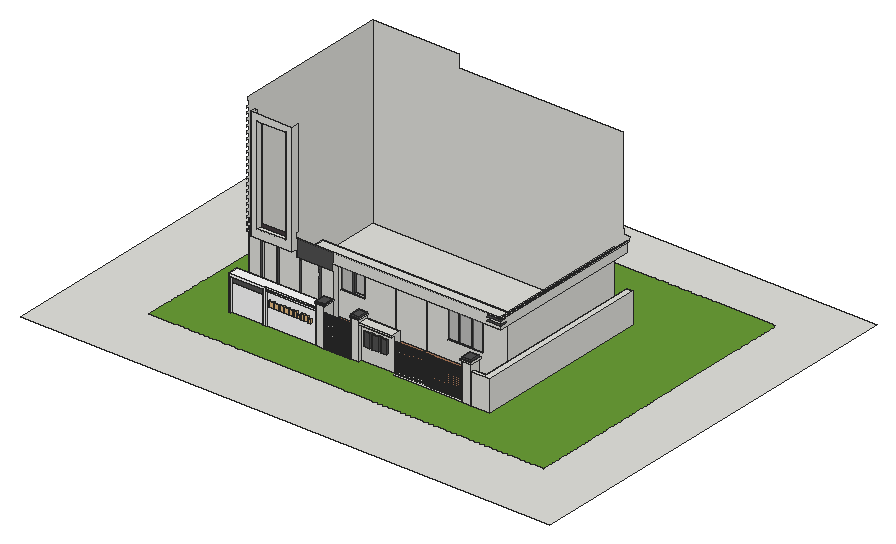
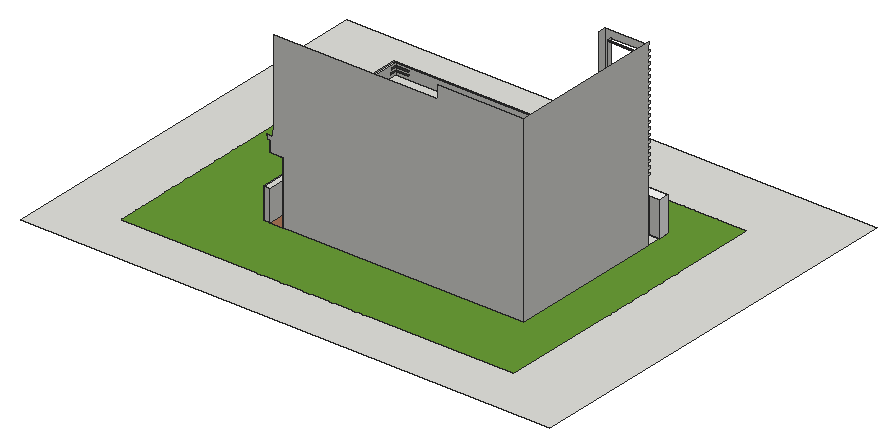
# SketchUp Ruby script. Lengths in inches.
U = 1.inch
M = Sketchup.active_model
def pt(a) = Geom::Point3d.new(a.map { |v| v * U })
def face(e, loops, mat)
  f = e.add_face(loops[0].map { |a| pt(a) })
  loops[1..].each { |l| e.add_face(l.map { |a| pt(a) }).erase! }
  f.material = f.back_material = mat if mat
  f
end
# faces: each face lists its corners as indices into pts; further lists are holes
def faces(e, pts, list, mat = nil) = list.each { |f| face(e, (f[0].is_a?(Array) ? f : [f]).map { |l| l.map { |i| pts[i] } }, mat) }
# xy, xz, yz: faces in a plane at the given z, y or x. An outline is a flat list of corners, or four numbers for a rectangle; further outlines are holes
def ring(l) = l.size == 4 ? [[l[0], l[1]], [l[2], l[1]], [l[2], l[3]], [l[0], l[3]]] : l.each_slice(2).to_a
def flat(e, list, mat, &to3) = list.each { |f| face(e, (f[0].is_a?(Array) ? f : [f]).map { |l| ring(l).map { |u, v| to3.(u, v) } }, mat) }
def xy(e, z, list, mat = nil) = flat(e, list, mat) { |x, y| [x, y, z] }
def xz(e, y, list, mat = nil) = flat(e, list, mat) { |x, z| [x, y, z] }
def yz(e, x, list, mat = nil) = flat(e, list, mat) { |y, z| [x, y, z] }
def lines(e, pts, list) = list.each { |a, b| e.add_line(pt(pts[a]), pt(pts[b])) }
# prism: a flat outline (further loops are holes) pulled along v
def prism(e, loops, v, mat = nil)
  f = face(e, loops, mat); d = Geom::Vector3d.new(v.map { |x| x * U })
  f.pushpull(f.normal.samedirection?(d) ? d.length : -d.length)
end
def box(e, o, s, mat = nil) = prism(e, [[o, [o[0] + s[0], o[1], o[2]], [o[0] + s[0], o[1] + s[1], o[2]], [o[0], o[1] + s[1], o[2]]]], [0, 0, s[2]], mat)
def at(x, y, z, deg = 0) = Geom::Transformation.translation(pt([x, y, z])) * Geom::Transformation.rotation(ORIGIN, Z_AXIS, deg.degrees)
def axes(o, x, y, z) = Geom::Transformation.new([*x, 0, *y, 0, *z, 0, *pt(o).to_a, 1])
def part(name) = M.definitions.add(name)
# library, detail: a bought-in or finely detailed component or shape, given as its bounding box
def library(name, o, s) = part(name).tap { |d| box(d.entities, o, s) }
def detail(e, o, s) = box(e.add_group.entities, o, s)
def put(e, d, t, mat = nil) = e.add_instance(d, t).tap { |i| i.material = mat if mat }
def group(e, t, mat = nil) = e.add_group.tap { |g| g.transformation = t; g.material = mat if mat }.entities
root = M.entities
M.materials.add("Color_008").color = [30, 30, 30]
M.materials.add("[0055_LightGoldenrodYellow]").color = [250, 250, 210]
M.materials.add("[0128_White]").color = [255, 255, 255]
M.materials.add("[0135_DarkGray]").color = [81, 81, 81]
M.materials.add("[Asphalt New]").color = [67, 60, 62]
M.materials.add("[Grass Dark Green]").color = [106, 157, 55]
M.materials.add("[Tile Ceramic Multi]").color = [165, 115, 84]
M.materials.add("[Translucent Glass Gray]").color = [128, 128, 128]
M.materials["[Translucent Glass Gray]"].alpha = 0.5
c1 = part("DOOR12")
g1 = group(c1.entities,at(114.73,28.14,-0.51))
g2 = group(g1,at(0,0,0))
box(g2,[0,0,0],[36,0.5,77.7])
c2 = part("Gate slat")
box(c2.entities,[0,0,-2.03],[1.97,0.97,40.94])
c3 = part("Gate frame upright")
box(c3.entities,[0,0,0],[1.9,0.97,93.54])
c4 = part("Group\#7")
p = [[41.47,0.97,43.31],[41.47,0.97,44.29]]
lines(c4.entities,p,[[0,1]])
put(c4.entities,c2,axes([3.81,0,13.78],[0,0,-1],[0,1,0],[0.96774,0,0]),"Color_008")
put(c4.entities,c2,axes([3.81,0,44.29],[0,0,-1],[0,1,0],[0.96774,0,0]),"Color_008")
put(c4.entities,c2,axes([47.12,0,9.84],[0,0,-1],[0,1,0],[0.96774,0,0]),"Color_008")
put(c4.entities,c2,axes([3.81,0,5.91],[0,0,-1],[0,1,0],[0.96774,0,0]),"Color_008")
put(c4.entities,c2,axes([3.81,0,17.72],[0,0,-1],[0,1,0],[0.96774,0,0]),"Color_008")
put(c4.entities,c2,axes([47.12,0,17.72],[0,0,-1],[0,1,0],[0.96774,0,0]),"Color_008")
put(c4.entities,c2,axes([47.12,0,5.91],[0,0,-1],[0,1,0],[0.96774,0,0]),"Color_008")
put(c4.entities,c2,axes([47.12,0,21.65],[0,0,-1],[0,1,0],[0.96774,0,0]),"Color_008")
put(c4.entities,c2,axes([47.12,0,49.7],[0,0,-1],[0,1,0],[0.96774,0,0]),"Color_008")
put(c4.entities,c2,axes([47.12,0,13.78],[0,0,-1],[0,1,0],[0.96774,0,0]),"Color_008")
put(c4.entities,c2,axes([47.12,0,44.29],[0,0,-1],[0,1,0],[0.96774,0,0]),"Color_008")
put(c4.entities,c2,axes([3.81,0,1.97],[0,0,-1],[0,1,0],[0.96774,0,0]),"Color_008")
put(c4.entities,c2,axes([47.12,0,38.88],[0,0,-1],[0,1,0],[0.96774,0,0]),"Color_008")
put(c4.entities,c2,axes([47.12,0,55.12],[0,0,-1],[0,1,0],[0.96774,0,0]),"Color_008")
put(c4.entities,c2,axes([3.81,0,9.84],[0,0,-1],[0,1,0],[0.96774,0,0]),"Color_008")
put(c4.entities,c2,axes([3.81,0,38.88],[0,0,-1],[0,1,0],[0.96774,0,0]),"Color_008")
put(c4.entities,c2,axes([47.12,0,1.97],[0,0,-1],[0,1,0],[0.96774,0,0]),"Color_008")
put(c4.entities,c2,axes([3.81,0,21.65],[0,0,-1],[0,1,0],[0.96774,0,0]),"Color_008")
put(c4.entities,c3,axes([84.77,0,0],[0.96774,0,0],[0,1,0],[0,0,0.92593]),"Color_008")
put(c4.entities,c3,axes([41.47,0,0],[0.96774,0,0],[0,1,0],[0,0,0.92593]),"Color_008")
put(c4.entities,c2,axes([47.12,0,86.61],[0,0,-1],[0,1,0],[0.96774,0,0]),"Color_008")
put(c4.entities,c3,axes([0,0,0],[0.96774,0,0],[0,1,0],[0,0,0.92593]),"Color_008")
put(c4.entities,c2,axes([47.12,0,82.68],[0,0,-1],[0,1,0],[0.96774,0,0]),"Color_008")
put(c4.entities,c2,axes([3.81,0,82.68],[0,0,-1],[0,1,0],[0.96774,0,0]),"Color_008")
put(c4.entities,c2,axes([47.12,0,78.74],[0,0,-1],[0,1,0],[0.96774,0,0]),"Color_008")
put(c4.entities,c2,axes([47.12,0,74.8],[0,0,-1],[0,1,0],[0.96774,0,0]),"Color_008")
put(c4.entities,c2,axes([3.81,0,49.7],[0,0,-1],[0,1,0],[0.96774,0,0]),"Color_008")
put(c4.entities,c3,axes([43.31,0,0],[0.96774,0,0],[0,1,0],[0,0,0.92593]),"Color_008")
put(c4.entities,c2,axes([3.81,0,86.61],[0,0,-1],[0,1,0],[0.96774,0,0]),"Color_008")
put(c4.entities,c2,axes([3.81,0,59.06],[0,0,-1],[0,1,0],[0.96774,0,0]),"Color_008")
put(c4.entities,c2,axes([3.81,0,70.87],[0,0,-1],[0,1,0],[0.96774,0,0]),"Color_008")
put(c4.entities,c2,axes([47.12,0,70.87],[0,0,-1],[0,1,0],[0.96774,0,0]),"Color_008")
put(c4.entities,c2,axes([47.12,0,59.06],[0,0,-1],[0,1,0],[0.96774,0,0]),"Color_008")
put(c4.entities,c2,axes([47.12,0,29.53],[0,0,-1],[0,1,0],[0.96774,0,0]),"Color_008")
put(c4.entities,c2,axes([47.12,0,62.99],[0,0,-1],[0,1,0],[0.96774,0,0]),"Color_008")
put(c4.entities,c2,axes([3.81,0,78.74],[0,0,-1],[0,1,0],[0.96774,0,0]),"Color_008")
put(c4.entities,c2,axes([3.81,0,33.46],[0,0,-1],[0,1,0],[0.96774,0,0]),"Color_008")
put(c4.entities,c2,axes([3.81,0,25.59],[0,0,-1],[0,1,0],[0.96774,0,0]),"Color_008")
put(c4.entities,c2,axes([47.12,0,25.59],[0,0,-1],[0,1,0],[0.96774,0,0]),"Color_008")
put(c4.entities,c2,axes([47.12,0,33.46],[0,0,-1],[0,1,0],[0.96774,0,0]),"Color_008")
put(c4.entities,c2,axes([3.81,0,66.93],[0,0,-1],[0,1,0],[0.96774,0,0]),"Color_008")
put(c4.entities,c2,axes([3.81,0,55.12],[0,0,-1],[0,1,0],[0.96774,0,0]),"Color_008")
put(c4.entities,c2,axes([3.81,0,74.8],[0,0,-1],[0,1,0],[0.96774,0,0]),"Color_008")
put(c4.entities,c2,axes([47.12,0,66.93],[0,0,-1],[0,1,0],[0.96774,0,0]),"Color_008")
put(c4.entities,c2,axes([3.81,0,62.99],[0,0,-1],[0,1,0],[0.96774,0,0]),"Color_008")
put(c4.entities,c2,axes([3.81,0,29.53],[0,0,-1],[0,1,0],[0.96774,0,0]),"Color_008")
c5 = part("Slatted gate assembly")
put(c5.entities,c4,axes([-88.13,609.51,-153.07],[1.3627,0,0],[0,1,0],[0,0,1.7688]))
put(c5.entities,c4,axes([217.15,626.41,-153.07],[3.6501,0,0],[0,1,0],[0,0,1.57423]))
c6 = part("Porton+casa")
put(c6.entities,c5,axes([-105.86,-50.18,-35.42],[0.96774,0,0],[0,1,0],[0,0,0.92]),"[0055_LightGoldenrodYellow]")
c7 = part("HOUSEdekho")
detail(c7.entities,[13.61,0,0],[122.37,130.74,27.32])
detail(c7.entities,[139.51,2.7,0],[109.26,119.35,27.32])
detail(c7.entities,[266.3125,3.93,0],[109.26,124.92,27.32])
detail(c7.entities,[374.26,1.97,0],[101.97,133.28,27.32])
detail(c7.entities,[480.41,2.38,0],[107.46,121.47,27.32])
detail(c7.entities,[578.2,6.07,0],[89.34,129.01,27.32])
detail(c7.entities,[670.57,4.75,0],[69.1,74.76,27.32])
detail(c7.entities,[753.93,3.6875,0],[74.84,122.38,27.32])
detail(c7.entities,[927.21,3.11,0],[75.49,84.19,27.32])
detail(c7.entities,[835.74,1.72,0],[78.19,128.28,27.32])
xy(root,0,[[[0,0,2325.4375,1794.125],[329.35,294.58,2062.92,1577.15]],[532.875,477.43,543.6,483.37],[684.29,477.43,695.02,483.37],[913.0625,479.97,913.0625,483.37,532.875,483.37,532.875,524.75,913.0625,524.75,913.0625,527.12,951.19,527.12,951.19,479.97],[951.19,483.37,1065.875,527.12],
  [1065.875,483.37,1065.875,527.12,1246.63,527.12,1246.63,496.87,1099.875,496.87,1099.875,483.37],[1246.63,483.37,1552.58,527.12],[1552.58,483.37,1589.25,527.12],[1589.25,483.37,1592.39,527.12],[532.875,524.75,579.8125,586.48],
  [532.875,586.48,532.875,1270.99,1589.25,1270.99,1589.25,688.36,1235.36,688.36,1235.36,717.42,1098.36,717.42,1098.36,688.36,778.18,688.36,778.18,603.86,910.24,603.86,910.24,586.48,658.4375,586.48,658.4375,591.23,594.625,591.23,594.625,586.48]])
xy(root,0,[[[329.35,294.58,2062.92,1577.15],[951.19,483.37,1099.875,483.37,1099.875,496.87,1246.63,496.87,1246.63,483.37,1592.39,483.37,1592.39,500.06,1645.64,500.06,1645.64,1270.99,532.875,1270.99,532.875,524.75,913.0625,524.75,913.0625,527.12,951.19,527.12],[684.29,477.43,695.02,483.37],[532.875,477.43,543.6,483.37]]],"[Grass Dark Green]")
xy(root,0,[[1592.39,500.06,1592.39,527.12,913.0625,527.12,913.0625,524.75,579.8125,524.75,579.8125,586.48,594.625,586.48,594.625,591.23,658.4375,591.23,658.4375,586.48,910.24,586.48,910.24,603.86,778.18,603.86,778.18,688.36,1098.36,688.36,1098.36,717.42,1235.36,717.42,1235.36,688.36,1589.25,688.36,1589.25,1270.99,1645.64,1270.99,1645.64,500.06]],"[Tile Ceramic Multi]")
xy(root,64.54,[[1117.42,489.06,1144.73,496.87],[1154.73,489.06,1182.04,496.87],[1191.48,489.06,1218.79,496.87]],"[0135_DarkGray]")
xy(root,110.86,[[917.5,688.36,964.04,698.67]],"[Translucent Glass Gray]")
xy(root,119.52,[[543.6,481,684.29,483.37]])
xy(root,122.73,[[1117.42,489.06,1144.73,496.87],[1154.73,489.06,1182.04,496.87],[1191.48,489.06,1218.79,496.87]],"[0135_DarkGray]")
xy(root,133.4375,[[1592.39,483.37,1674.21,483.37,1674.21,1270.99,1645.64,1270.99,1645.64,500.06,1592.39,500.06]])
xy(root,136.09,[[695.02,479.97,913.0625,483.37]])
xy(root,141.43,[[695.02,479.97,913.0625,483.37]],"[0128_White]")
xy(root,141.65,[[543.6,477.43,684.29,481]])
xy(root,146.34,[[1099.875,483.37,1246.63,496.87]])
xy(root,146.6,[[695.02,479.97,913.0625,483.37]],"[0128_White]")
xy(root,152.375,[[1099.875,483.37,1246.63,527.12]])
xy(root,152.375,[[532.875,477.43,532.875,524.75,913.0625,524.75,913.0625,479.97,695.02,479.97,695.02,477.43]],"[0128_White]")
xy(root,165.3125,[[909.66,479.97,913.0625,479.97,913.0625,527.12,951.19,527.12,951.19,479.97,954.6,479.97,954.6,530.52,909.66,530.52],[913.0625,479.97,951.19,483.37]])
xy(root,165.375,[[[1547.82,478.61,1597.15,531.88],[1552.58,483.37,1592.39,527.12]],[[1062.44,479.9375,1103.3,530.55],[1065.875,483.37,1099.875,527.12]]])
xy(root,169.6875,[[[909.66,479.97,954.6,530.52],[913.0625,483.37,951.19,527.12]]],"[0128_White]")
xy(root,169.75,[[[1062.44,479.9375,1103.3,530.55],[1065.875,483.37,1099.875,527.12]]])
xy(root,169.9375,[[[1547.82,478.61,1597.15,531.88],[1552.58,483.37,1592.39,527.12]]])
xy(root,174.6875,[[913.0625,483.37,951.19,527.12]],"[0135_DarkGray]")
xy(root,175.5,[[1065.875,483.37,1099.875,527.12]],"[0135_DarkGray]")
xy(root,178.625,[[1552.58,483.37,1592.39,527.12]],"[0135_DarkGray]")
xy(root,235.54,[[917.5,688.36,964.04,698.67]],"[Translucent Glass Gray]")
xy(root,242.5625,[[1098.36,688.36,1235.36,717.42]])
xy(root,247.92,[[749.43,579.23,910.24,586.48]])
xy(root,272.9,[[532.875,579.23,567.67,586.48],[567.67,579.23,567.67,586.48,594.625,586.48,594.625,591.23,658.4375,591.23,658.4375,586.48,749.43,586.48,749.43,579.23]])
xy(root,275.86,[[567.67,556.73,749.43,579.23],[910.24,579.23,910.24,603.86,778.18,603.86,778.18,688.36,1589.25,688.36,1589.25,625.42,1647.5625,625.42,1647.5625,579.23],[1589.25,625.42,1647.5625,657.42],[1589.25,657.42,1647.5625,1270.99]])
xy(root,282.63,[[532.875,579.23,567.67,588.61]])
xy(root,298.46,[[532.875,578.55,567.67,588.61]])
xy(root,308.19,[[532.875,578.55,567.67,588.61]])
xy(root,314.18,[[595.83,556.73,721.27,575.61]])
xy(root,322.85,[[749.43,575.61,1658.1875,579.23],[1647.5625,579.23,1658.1875,1270.99]])
xz(root,477.43,[[532.875,0,532.875,152.375,695.02,152.375,695.02,0,684.29,0,684.29,141.65,543.6,141.65,543.6,0]],"[0128_White]")
xz(root,478.61,[[1547.82,165.375,1597.15,169.9375]])
xz(root,479.9375,[[1062.44,165.375,1103.3,169.75]])
xz(root,479.97,[[913.0625,0,951.19,165.3125]])
xz(root,479.97,[[695.02,136.09,913.0625,141.43],[695.02,146.6,913.0625,152.375],[909.66,165.3125,954.6,169.6875]],"[0128_White]")
xz(root,481,[[543.6,119.52,684.29,141.65]],"[0135_DarkGray]")
xz(root,483.37,[[1065.875,0,1099.875,165.375],[1552.58,0,1592.39,165.375],[1592.39,0,1674.21,133.4375],[1099.875,146.34,1246.63,152.375],[913.0625,165.3125,951.19,169.6875],
  [1065.875,165.375,1099.875,169.75],[1552.58,165.375,1592.39,169.9375]])
xz(root,483.37,[[543.6,0,684.29,119.52],[695.02,0,913.0625,136.09]],"[0128_White]")
xz(root,483.37,[[695.02,141.43,913.0625,146.6],[913.0625,169.6875,951.19,174.6875],[1065.875,169.75,1099.875,175.5],[1552.58,169.9375,1592.39,178.625]],"[0135_DarkGray]")
xz(root,489.06,[[1117.42,64.54,1144.73,122.73],[1154.73,64.54,1182.04,122.73],[1191.48,64.54,1218.79,122.73]],"[0135_DarkGray]")
xz(root,496.87,[[[1099.875,0,1246.63,146.34],[1117.42,64.54,1144.73,122.73],[1154.73,64.54,1182.04,122.73],[1191.48,64.54,1218.79,122.73]]])
xz(root,500.06,[[1592.39,0,1645.64,133.4375]])
xz(root,524.75,[[532.875,0,579.8125,152.375],[579.8125,0,913.0625,152.375]])
xz(root,527.12,[[913.0625,0,951.19,165.3125],[1065.875,0,1099.875,169.75],[1099.875,0,1246.63,152.375],[1552.58,0,1592.39,165.375],[913.0625,165.3125,951.19,169.6875],
  [1552.58,165.375,1592.39,169.9375],[913.0625,169.6875,951.19,174.6875],[1065.875,169.75,1099.875,175.5],[1552.58,169.9375,1592.39,178.625]])
xz(root,530.52,[[909.66,165.3125,954.6,169.6875]])
xz(root,530.55,[[1062.44,165.375,1103.3,169.75]])
xz(root,531.88,[[1547.82,165.375,1597.15,169.9375]])
xz(root,556.73,[[[567.67,275.86,749.43,766.13],[595.83,314.18,721.27,737.97]]])
xz(root,575.61,[[749.43,322.85,1658.1875,325.125]])
xz(root,575.61,[[[595.83,314.18,721.27,737.97],[600.1,327.45,716.99,733.69]]],"[Asphalt New]")
xz(root,578.55,[[532.875,298.46,567.67,308.19]])
xz(root,579.23,[[532.875,272.9,749.43,272.9,749.43,275.86,567.67,275.86,567.67,282.63,532.875,282.63],[910.24,275.86,1647.5625,275.86,1647.5625,288.68,1586.625,288.68,1586.625,297.37,1647.5625,297.37,1647.5625,304.87,1585.9375,304.87,1585.9375,315.18,1647.5625,315.18,1647.5625,322.85,910.24,322.85]])
xz(root,579.23,[[749.43,247.92,910.24,322.85],[1586.625,288.68,1647.5625,297.37],[1585.9375,304.87,1647.5625,315.18]],"[0135_DarkGray]")
xz(root,586.48,[[532.875,0,583.75,272.9],[669.3125,0,754.25,0,754.25,247.92,749.43,247.92,749.43,272.9,669.3125,272.9],[765.125,0,842.5625,247.92],[853.4375,0,910.24,247.92]])
xz(root,586.48,[[583.75,0,594.625,272.9],[658.4375,0,669.3125,272.9],[754.25,0,765.125,247.92],[842.5625,0,853.4375,247.92]],"[0135_DarkGray]")
xz(root,588.61,[[532.875,282.63,567.67,298.46],[532.875,308.19,567.67,324.03]],"[0135_DarkGray]")
xz(root,591.23,[[594.625,0,658.4375,272.9]])
xz(root,603.86,[[778.18,0,910.24,275.86]])
xz(root,688.36,[[[778.18,0,1098.36,0,1098.36,242.5625,1235.36,242.5625,1235.36,0,1589.25,0,1589.25,275.86,778.18,275.86],[1329.36,75.69,1486.79,226.45],[856.42,107.36,967.55,239.05]]])
xz(root,688.36,[[[856.42,107.36,967.55,239.05],[859.92,110.86,964.04,235.54]],[911.98,110.86,917.5,235.54]],"[0135_DarkGray]")
xz(root,688.36,[[[1329.36,75.69,1486.79,226.45],[1333.49,79.82,1482.67,222.32]],[1374.76,79.82,1378.91,222.32],[1430.79,79.82,1435.48,222.32]],"[Asphalt New]")
xz(root,688.36,[[1333.49,79.82,1374.76,222.32],[1378.91,79.82,1430.79,222.32],[1435.48,79.82,1482.67,222.32],[859.92,110.86,911.98,235.54]],"[Translucent Glass Gray]")
xz(root,698.67,[[917.5,110.86,964.04,235.54]],"[Translucent Glass Gray]")
xz(root,717.42,[[1098.36,0,1235.36,242.5625]])
xz(root,1270.99,[[532.875,0,532.875,799.9375,910.24,799.9375,910.24,745.125,1630.5,745.125,1630.5,365.875,1634.625,365.875,1634.625,342.73,1660.625,342.73,1660.625,338.38,1655,338.38,1655,325.125,1658.1875,325.125,1658.1875,322.85,1647.5625,322.85,1647.5625,275.86,1589.25,275.86,1589.25,0],[1645.64,0,1674.21,133.4375]])
yz(root,532.875,[[586.48,0,586.48,272.9,579.23,272.9,579.23,282.63,588.61,282.63,588.61,298.46,578.55,298.46,578.55,308.19,588.61,308.19,588.61,324.03,578.55,324.03,578.55,333.75,588.61,333.75,588.61,349.59,578.55,349.59,578.55,359.32,588.61,359.32,588.61,375.15,578.55,375.15,578.55,384.88,588.61,384.88,588.61,400.71,578.55,400.71,578.55,410.44,588.61,410.44,588.61,426.28,578.55,426.28,578.55,436,588.61,436,588.61,451.84,578.55,451.84,578.55,461.57,588.61,461.57,588.61,477.4,578.55,477.4,578.55,487.13,588.61,487.13,588.61,502.96,578.55,502.96,578.55,512.69,588.61,512.69,588.61,528.53,578.55,528.53,578.55,538.25,588.61,538.25,588.61,554.09,578.55,554.09,578.55,563.82,588.61,563.82,588.61,579.65,578.55,579.65,578.55,589.38,588.61,589.38,588.61,605.21,578.55,605.21,578.55,614.94,588.61,614.94,588.61,630.78,578.55,630.78,578.55,640.5,588.61,640.5,588.61,656.34,578.55,656.34,578.55,666.07,588.61,666.07,588.61,681.9,578.55,681.9,578.55,691.63,588.61,691.63,588.61,707.46,578.55,707.46,578.55,717.19,588.61,717.19,588.61,733.03,578.55,733.03,578.55,742.75,588.61,742.75,588.61,756.4,578.55,756.4,578.55,766.13,588.61,766.13,588.61,786.75,583.8,786.75,583.8,799.9375,1270.99,799.9375,1270.99,0]])
yz(root,532.875,[[477.43,0,524.75,152.375]],"[0128_White]")
yz(root,543.6,[[477.43,0,477.43,141.65,481,141.65,481,119.52,483.37,119.52,483.37,0]],"[0128_White]")
yz(root,567.67,[[556.73,275.86,556.73,766.13,578.55,766.13,578.55,756.4,588.61,756.4,588.61,742.75,578.55,742.75,578.55,733.03,588.61,733.03,588.61,717.19,578.55,717.19,578.55,707.46,588.61,707.46,588.61,691.63,578.55,691.63,578.55,681.9,588.61,681.9,588.61,666.07,578.55,666.07,578.55,656.34,588.61,656.34,588.61,640.5,578.55,640.5,578.55,630.78,588.61,630.78,588.61,614.94,578.55,614.94,578.55,605.21,588.61,605.21,588.61,589.38,578.55,589.38,578.55,579.65,588.61,579.65,588.61,563.82,578.55,563.82,578.55,554.09,588.61,554.09,588.61,538.25,578.55,538.25,578.55,528.53,588.61,528.53,588.61,512.69,578.55,512.69,578.55,502.96,588.61,502.96,588.61,487.13,578.55,487.13,578.55,477.4,588.61,477.4,588.61,461.57,578.55,461.57,578.55,451.84,588.61,451.84,588.61,436,578.55,436,578.55,426.28,588.61,426.28,588.61,410.44,578.55,410.44,578.55,400.71,588.61,400.71,588.61,384.88,578.55,384.88,578.55,375.15,588.61,375.15,588.61,359.32,578.55,359.32,578.55,349.59,588.61,349.59,588.61,333.75,578.55,333.75,578.55,324.03,588.61,324.03,588.61,308.19,578.55,308.19,578.55,298.46,588.61,298.46,588.61,282.63,579.23,282.63,579.23,275.86]])
yz(root,594.625,[[586.48,0,591.23,272.9]])
yz(root,595.83,[[556.73,314.18,575.61,737.97]])
yz(root,658.4375,[[586.48,0,591.23,272.9]])
yz(root,684.29,[[477.43,0,483.37,0,483.37,119.52,481,119.52,481,141.65,477.43,141.65]],"[0128_White]")
yz(root,695.02,[[477.43,0,477.43,152.375,479.97,152.375,479.97,146.6,483.37,146.6,483.37,141.43,479.97,141.43,479.97,136.09,483.37,136.09,483.37,0]],"[0128_White]")
yz(root,721.27,[[556.73,314.18,575.61,737.97]])
yz(root,749.43,[[579.23,247.92,586.48,272.9],[556.73,275.86,579.23,275.86,579.23,322.85,575.61,322.85,575.61,325.125,578.42,325.125,578.42,338.38,573.8,338.38,573.8,342.73,588.61,342.73,588.61,766.13,556.73,766.13]])
yz(root,778.18,[[603.86,0,688.36,275.86]])
yz(root,909.66,[[479.97,165.3125,524.75,169.6875],[524.75,165.3125,530.52,169.6875]],"[0128_White]")
yz(root,910.24,[[586.48,0,603.86,0,603.86,275.86,579.23,275.86,579.23,247.92,586.48,247.92]])
yz(root,913.0625,[[479.97,0,483.37,136.09],[524.75,0,527.12,165.3125],[479.97,141.43,483.37,146.6],[479.97,152.375,524.75,165.3125],[483.37,165.3125,524.75,169.6875],
  [524.75,165.3125,527.12,169.6875],[524.75,169.6875,527.12,174.6875]])
yz(root,913.0625,[[483.37,169.6875,524.75,174.6875]],"[0135_DarkGray]")
yz(root,917.5,[[688.36,110.86,698.67,235.54]],"[Translucent Glass Gray]")
yz(root,951.19,[[479.97,0,527.12,165.3125],[483.37,165.3125,527.12,169.6875]])
yz(root,951.19,[[483.37,169.6875,527.12,174.6875]],"[0135_DarkGray]")
yz(root,954.6,[[479.97,165.3125,530.52,169.6875]])
yz(root,964.04,[[688.36,110.86,698.67,235.54]],"[Translucent Glass Gray]")
yz(root,1062.44,[[479.9375,165.375,530.55,169.75]])
yz(root,1065.875,[[483.37,0,527.12,169.75]])
yz(root,1065.875,[[483.37,169.75,527.12,175.5]],"[0135_DarkGray]")
yz(root,1098.36,[[688.36,0,717.42,242.5625]])
yz(root,1099.875,[[483.37,0,496.87,146.34],[483.37,152.375,527.12,169.75]])
yz(root,1099.875,[[483.37,169.75,527.12,175.5]],"[0135_DarkGray]")
yz(root,1103.3,[[479.9375,165.375,530.55,169.75]])
yz(root,1117.42,[[489.06,64.54,496.87,122.73]])
yz(root,1144.73,[[489.06,64.54,496.87,122.73]],"[0135_DarkGray]")
yz(root,1154.73,[[489.06,64.54,496.87,122.73]],"[0135_DarkGray]")
yz(root,1182.04,[[489.06,64.54,496.87,122.73]],"[0135_DarkGray]")
yz(root,1191.48,[[489.06,64.54,496.87,122.73]],"[0135_DarkGray]")
yz(root,1218.79,[[489.06,64.54,496.87,122.73]],"[0135_DarkGray]")
yz(root,1235.36,[[688.36,0,717.42,242.5625]])
yz(root,1246.63,[[496.87,0,527.12,0,527.12,152.375,483.37,152.375,483.37,146.34,496.87,146.34]])
yz(root,1547.82,[[478.61,165.375,531.88,169.9375]])
yz(root,1552.58,[[483.37,0,527.12,169.9375]])
yz(root,1552.58,[[483.37,169.9375,527.12,178.625]],"[0135_DarkGray]")
yz(root,1589.25,[[688.36,0,1270.99,275.86]])
yz(root,1592.39,[[483.37,0,500.06,133.4375],[500.06,0,527.12,81.9375],[500.06,81.9375,527.12,81.9375,527.12,165.375,483.37,165.375,483.37,133.4375,500.06,133.4375],[483.37,165.375,527.12,169.9375]])
yz(root,1592.39,[[483.37,169.9375,527.12,178.625]],"[0135_DarkGray]")
yz(root,1597.15,[[478.61,165.375,531.88,169.9375]])
yz(root,1645.64,[[500.06,0,1270.99,133.4375]])
yz(root,1647.5625,[[579.23,275.86,1270.99,275.86,1270.99,322.85,579.23,322.85,579.23,315.18,607.55,315.18,607.55,305.25,579.23,305.25,579.23,297.37,612.11,297.37,612.11,288.68,579.23,288.68]])
yz(root,1647.5625,[[579.23,288.68,612.11,297.37],[579.23,305.25,607.55,315.18]],"[0135_DarkGray]")
yz(root,1658.1875,[[575.61,322.85,1270.99,325.125]])
yz(root,1674.21,[[483.37,0,1270.99,133.4375]])
p = [[765.125,586.48,272.9],[765.125,586.48,247.92],[754.25,586.48,247.92],[754.25,586.48,272.9],[853.4375,586.48,272.9],[853.4375,586.48,247.92],
  [842.5625,586.48,247.92],[842.5625,586.48,272.9]]
lines(root,p,[[0,1],[2,3],[4,5],[6,7]])
put(root,c1,axes([659.51,599.07,1.6],[3.82519,0,0],[0,3.1354,0],[0,0,3.1354]))
put(root,c6,at(1142.35,-79.36,176.24))
put(root,c7,axes([705.27,483.37,79.06],[0.19,0,0],[0,0,0.19],[0,-0.19,0]))
